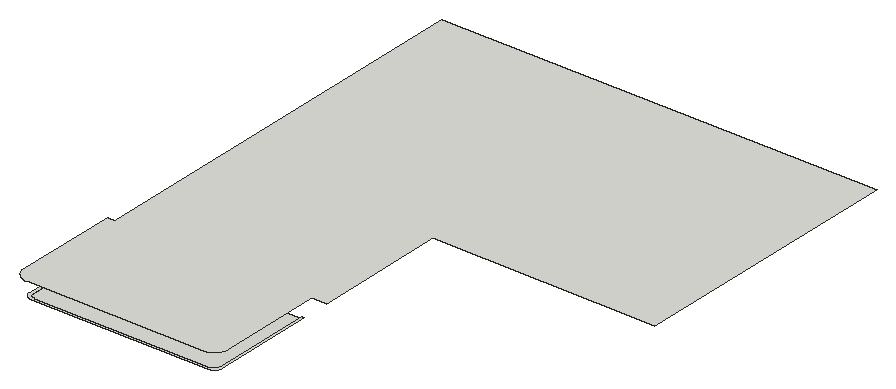
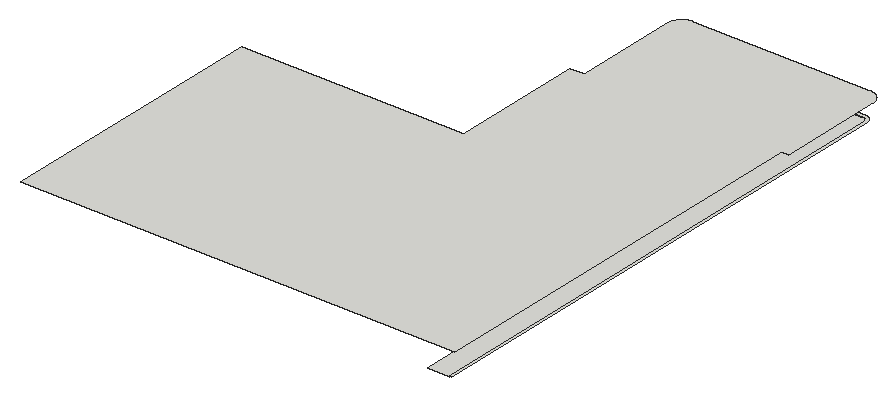
# SketchUp Ruby script. Lengths in inches.
U = 1.inch
M = Sketchup.active_model
def pt(a) = Geom::Point3d.new(a.map { |v| v * U })
def face(e, loops, mat)
  f = e.add_face(loops[0].map { |a| pt(a) })
  loops[1..].each { |l| e.add_face(l.map { |a| pt(a) }).erase! }
  f.material = f.back_material = mat if mat
  f
end
# faces: each face lists its corners as indices into pts; further lists are holes
def faces(e, pts, list, mat = nil) = list.each { |f| face(e, (f[0].is_a?(Array) ? f : [f]).map { |l| l.map { |i| pts[i] } }, mat) }
# xy, xz, yz: faces in a plane at the given z, y or x. An outline is a flat list of corners, or four numbers for a rectangle; further outlines are holes
def ring(l) = l.size == 4 ? [[l[0], l[1]], [l[2], l[1]], [l[2], l[3]], [l[0], l[3]]] : l.each_slice(2).to_a
def flat(e, list, mat, &to3) = list.each { |f| face(e, (f[0].is_a?(Array) ? f : [f]).map { |l| ring(l).map { |u, v| to3.(u, v) } }, mat) }
def xy(e, z, list, mat = nil) = flat(e, list, mat) { |x, y| [x, y, z] }
def xz(e, y, list, mat = nil) = flat(e, list, mat) { |x, z| [x, y, z] }
def yz(e, x, list, mat = nil) = flat(e, list, mat) { |y, z| [x, y, z] }
def lines(e, pts, list) = list.each { |a, b| e.add_line(pt(pts[a]), pt(pts[b])) }
# prism: a flat outline (further loops are holes) pulled along v
def prism(e, loops, v, mat = nil)
  f = face(e, loops, mat); d = Geom::Vector3d.new(v.map { |x| x * U })
  f.pushpull(f.normal.samedirection?(d) ? d.length : -d.length)
end
def box(e, o, s, mat = nil) = prism(e, [[o, [o[0] + s[0], o[1], o[2]], [o[0] + s[0], o[1] + s[1], o[2]], [o[0], o[1] + s[1], o[2]]]], [0, 0, s[2]], mat)
def at(x, y, z, deg = 0) = Geom::Transformation.translation(pt([x, y, z])) * Geom::Transformation.rotation(ORIGIN, Z_AXIS, deg.degrees)
def axes(o, x, y, z) = Geom::Transformation.new([*x, 0, *y, 0, *z, 0, *pt(o).to_a, 1])
def part(name) = M.definitions.add(name)
# library, detail: a bought-in or finely detailed component or shape, given as its bounding box
def library(name, o, s) = part(name).tap { |d| box(d.entities, o, s) }
def detail(e, o, s) = box(e.add_group.entities, o, s)
def put(e, d, t, mat = nil) = e.add_instance(d, t).tap { |i| i.material = mat if mat }
def group(e, t, mat = nil) = e.add_group.tap { |g| g.transformation = t; g.material = mat if mat }.entities
root = M.entities
xy(root,247,[[[29.8,234,29.74,234.01,29.67,234.01,29.61,234.02,29.54,234.02,29.48,234.03,29.41,234.03,29.35,234.04,29.28,234.05,29.22,234.0625,29.15,234.07,29.09,234.08,29.02,234.1,28.96,234.11,28.9,234.125,28.83,234.14,28.77,234.15,28.71,234.17,28.64,234.1875,28.58,234.21,28.52,234.22,28.45,234.24,28.39,234.27,28.21,234.33,28.15,234.36,28.09,234.38,28.03,234.41,27.97,234.43,27.79,234.52,27.73,234.54,27.67,234.58,27.61,234.61,27.56,234.64,27.44,234.7,27.39,234.74,27.33,234.77,27.28,234.81,27.22,234.84,27.17,234.88,27.11,234.92,27.0625,234.95,27.01,234.99,26.96,235.03,26.9,235.07,26.85,235.11,26.8,235.16,26.65,235.28,26.61,235.33,26.51,235.42,26.46,235.46,26.42,235.51,26.33,235.61,26.28,235.65,26.16,235.8,26.11,235.85,26.07,235.9,26.03,235.96,25.99,236.01,25.95,236.0625,25.92,236.11,25.88,236.17,25.84,236.22,25.81,236.28,25.77,236.33,25.74,236.39,25.7,236.44,25.64,236.56,25.61,236.61,25.58,236.67,25.54,236.73,25.52,236.79,25.43,236.97,25.41,237.03,25.38,237.09,25.36,237.15,25.33,237.21,25.27,237.39,25.24,237.45,25.22,237.52,25.21,237.58,25.1875,237.64,25.17,237.71,25.15,237.77,25.14,237.83,25.125,237.9,25.11,237.96,25.1,238.02,25.08,238.09,25.07,238.15,25.0625,238.22,25.05,238.28,25.04,238.35,25.03,238.41,25.03,238.48,25.02,238.54,25.02,238.61,25.01,238.67,25.01,238.74,25,238.8,25,672,43,672,43,323.75,182,323.75,182,238.8,181.99,238.74,181.99,238.67,181.98,238.61,181.98,238.54,181.97,238.48,181.97,238.41,181.96,238.35,181.95,238.28,181.9375,238.22,181.93,238.15,181.92,238.09,181.9,238.02,181.89,237.96,181.875,237.9,181.86,237.83,181.85,237.77,181.83,237.71,181.8125,237.64,181.79,237.58,181.78,237.52,181.76,237.45,181.73,237.39,181.67,237.21,181.64,237.15,181.62,237.09,181.59,237.03,181.57,236.97,181.48,236.79,181.46,236.73,181.42,236.67,181.39,236.61,181.36,236.56,181.3,236.44,181.26,236.39,181.23,236.33,181.19,236.28,181.16,236.22,181.12,236.17,181.08,236.11,181.05,236.0625,181.01,236.01,180.97,235.96,180.93,235.9,180.89,235.85,180.84,235.8,180.72,235.65,180.67,235.61,180.58,235.51,180.54,235.46,180.49,235.42,180.39,235.33,180.35,235.28,180.2,235.16,180.15,235.11,180.1,235.07,180.04,235.03,179.99,234.99,179.9375,234.95,179.89,234.92,179.83,234.88,179.78,234.84,179.72,234.81,179.67,234.77,179.61,234.74,179.56,234.7,179.44,234.64,179.39,234.61,179.33,234.58,179.27,234.54,179.21,234.52,179.03,234.43,178.97,234.41,178.91,234.38,178.85,234.36,178.79,234.33,178.61,234.27,178.55,234.24,178.48,234.22,178.42,234.21,178.36,234.1875,178.29,234.17,178.23,234.15,178.17,234.14,178.1,234.125,178.04,234.11,177.98,234.1,177.91,234.08,177.85,234.07,177.78,234.0625,177.72,234.05,177.65,234.04,177.59,234.03,177.52,234.03,177.46,234.02,177.39,234.02,177.33,234.01,177.26,234.01,177.2,234],[103.34,272.75,103.66,272.75,103.74,272.76,103.8125,272.77,103.89,272.78,104.05,272.8,104.125,272.82,104.2,272.83,104.28,272.85,104.35,272.875,104.43,272.9,104.5,272.92,104.58,272.95,104.79,273.04,104.86,273.08,104.93,273.11,105.07,273.19,105.13,273.23,105.2,273.28,105.26,273.32,105.33,273.37,105.57,273.57,105.62,273.63,105.68,273.68,105.88,273.92,105.93,273.99,105.97,274.05,106.02,274.12,106.06,274.18,106.14,274.32,106.17,274.39,106.21,274.46,106.3,274.67,106.33,274.75,106.35,274.82,106.375,274.9,106.4,274.97,106.42,275.05,106.43,275.125,106.45,275.2,106.47,275.36,106.48,275.4375,106.49,275.51,106.5,275.59,106.5,275.91,106.49,275.99,106.48,276.0625,106.47,276.14,106.45,276.3,106.43,276.375,106.42,276.45,106.4,276.53,106.375,276.6,106.35,276.68,106.33,276.75,106.3,276.83,106.21,277.04,106.17,277.11,106.14,277.18,106.06,277.32,106.02,277.38,105.97,277.45,105.93,277.51,105.88,277.58,105.68,277.82,105.62,277.87,105.57,277.93,105.33,278.13,105.26,278.18,105.2,278.22,105.13,278.27,105.07,278.31,104.93,278.39,104.86,278.42,104.79,278.46,104.58,278.55,104.5,278.58,104.43,278.6,104.35,278.625,104.28,278.65,104.2,278.67,104.125,278.68,104.05,278.7,103.89,278.72,103.8125,278.73,103.74,278.74,103.66,278.75,103.34,278.75,103.26,278.74,103.1875,278.73,103.11,278.72,102.95,278.7,102.875,278.68,102.8,278.67,102.72,278.65,102.65,278.625,102.57,278.6,102.5,278.58,102.42,278.55,102.21,278.46,102.14,278.42,102.07,278.39,101.93,278.31,101.87,278.27,101.8,278.22,101.74,278.18,101.67,278.13,101.43,277.93,101.38,277.87,101.32,277.82,101.12,277.58,101.07,277.51,101.03,277.45,100.98,277.38,100.94,277.32,100.86,277.18,100.83,277.11,100.79,277.04,100.7,276.83,100.67,276.75,100.65,276.68,100.625,276.6,100.6,276.53,100.58,276.45,100.57,276.375,100.55,276.3,100.53,276.14,100.52,276.0625,100.51,275.99,100.5,275.91,100.5,275.59,100.51,275.51,100.52,275.4375,100.53,275.36,100.55,275.2,100.57,275.125,100.58,275.05,100.6,274.97,100.625,274.9,100.65,274.82,100.67,274.75,100.7,274.67,100.79,274.46,100.83,274.39,100.86,274.32,100.94,274.18,100.98,274.12,101.03,274.05,101.07,273.99,101.12,273.92,101.32,273.68,101.38,273.63,101.43,273.57,101.67,273.37,101.74,273.32,101.8,273.28,101.87,273.23,101.93,273.19,102.07,273.11,102.14,273.08,102.21,273.04,102.42,272.95,102.5,272.92,102.57,272.9,102.65,272.875,102.72,272.85,102.8,272.83,102.875,272.82,102.95,272.8,103.11,272.78,103.1875,272.77,103.26,272.76],[150.79,272.75,151.1,272.75,151.34,272.78,151.41,272.79,151.49,272.8,151.57,272.82,151.65,272.83,151.72,272.85,151.8,272.875,151.87,272.9,151.95,272.92,152.09,272.98,152.17,273.01,152.24,273.04,152.31,273.08,152.375,273.11,152.45,273.15,152.51,273.19,152.58,273.23,152.64,273.28,152.71,273.32,153.01,273.57,153.12,273.68,153.17,273.74,153.23,273.8,153.33,273.92,153.37,273.99,153.42,274.05,153.46,274.12,153.5,274.18,153.62,274.39,153.65,274.46,153.6875,274.53,153.72,274.6,153.75,274.67,153.77,274.75,153.8,274.82,153.82,274.9,153.84,274.97,153.86,275.05,153.88,275.125,153.89,275.2,153.91,275.28,153.92,275.36,153.93,275.4375,153.9375,275.51,153.94,275.59,153.94,275.67,153.95,275.75,153.94,275.83,153.94,275.91,153.9375,275.99,153.93,276.0625,153.92,276.14,153.91,276.22,153.89,276.3,153.88,276.375,153.86,276.45,153.84,276.53,153.82,276.6,153.8,276.68,153.77,276.75,153.75,276.83,153.72,276.9,153.6875,276.97,153.65,277.04,153.62,277.11,153.5,277.32,153.46,277.38,153.42,277.45,153.37,277.51,153.33,277.58,153.23,277.7,153.17,277.76,153.12,277.82,153.01,277.93,152.71,278.18,152.64,278.22,152.58,278.27,152.51,278.31,152.45,278.35,152.375,278.39,152.31,278.42,152.24,278.46,152.17,278.49,152.09,278.52,151.95,278.58,151.87,278.6,151.8,278.625,151.72,278.65,151.65,278.67,151.57,278.68,151.49,278.7,151.41,278.71,151.34,278.72,151.1,278.75,150.79,278.75,150.55,278.72,150.48,278.71,150.4,278.7,150.32,278.68,150.24,278.67,150.17,278.65,150.09,278.625,150.02,278.6,149.94,278.58,149.73,278.49,149.65,278.46,149.58,278.42,149.51,278.39,149.45,278.35,149.38,278.31,149.3125,278.27,149.25,278.22,149.18,278.18,149,278.03,148.9375,277.98,148.88,277.93,148.77,277.82,148.72,277.76,148.66,277.7,148.61,277.64,148.57,277.58,148.52,277.51,148.47,277.45,148.43,277.38,148.39,277.32,148.27,277.11,148.24,277.04,148.2,276.97,148.14,276.83,148.12,276.75,148.09,276.68,148.07,276.6,148.05,276.53,148.03,276.45,148.01,276.375,148,276.3,147.98,276.22,147.97,276.14,147.96,276.0625,147.95,275.99,147.95,275.51,147.96,275.4375,147.97,275.36,147.98,275.28,148,275.2,148.01,275.125,148.03,275.05,148.05,274.97,148.07,274.9,148.09,274.82,148.12,274.75,148.14,274.67,148.2,274.53,148.24,274.46,148.27,274.39,148.39,274.18,148.43,274.12,148.47,274.05,148.52,273.99,148.57,273.92,148.61,273.86,148.66,273.8,148.72,273.74,148.77,273.68,148.88,273.57,148.9375,273.52,149,273.47,149.18,273.32,149.25,273.28,149.3125,273.23,149.38,273.19,149.45,273.15,149.51,273.11,149.58,273.08,149.65,273.04,149.73,273.01,149.94,272.92,150.02,272.9,150.09,272.875,150.17,272.85,150.24,272.83,150.32,272.82,150.4,272.8,150.48,272.79,150.55,272.78],[55.9,272.75,56.21,272.75,56.45,272.78,56.52,272.79,56.6,272.8,56.68,272.82,56.76,272.83,56.83,272.85,56.91,272.875,56.98,272.9,57.06,272.92,57.27,273.01,57.35,273.04,57.42,273.08,57.49,273.11,57.55,273.15,57.62,273.19,57.6875,273.23,57.75,273.28,57.82,273.32,58,273.47,58.0625,273.52,58.12,273.57,58.23,273.68,58.28,273.74,58.34,273.8,58.39,273.86,58.43,273.92,58.48,273.99,58.53,274.05,58.57,274.12,58.61,274.18,58.73,274.39,58.76,274.46,58.8,274.53,58.86,274.67,58.88,274.75,58.91,274.82,58.93,274.9,58.95,274.97,58.97,275.05,58.99,275.125,59,275.2,59.02,275.28,59.03,275.36,59.04,275.4375,59.05,275.51,59.05,275.99,59.04,276.0625,59.03,276.14,59.02,276.22,59,276.3,58.99,276.375,58.97,276.45,58.95,276.53,58.93,276.6,58.91,276.68,58.88,276.75,58.86,276.83,58.8,276.97,58.76,277.04,58.73,277.11,58.61,277.32,58.57,277.38,58.53,277.45,58.48,277.51,58.43,277.58,58.39,277.64,58.34,277.7,58.28,277.76,58.23,277.82,58.12,277.93,58.0625,277.98,58,278.03,57.82,278.18,57.75,278.22,57.6875,278.27,57.62,278.31,57.55,278.35,57.49,278.39,57.42,278.42,57.35,278.46,57.27,278.49,57.06,278.58,56.98,278.6,56.91,278.625,56.83,278.65,56.76,278.67,56.68,278.68,56.6,278.7,56.52,278.71,56.45,278.72,56.21,278.75,55.9,278.75,55.66,278.72,55.59,278.71,55.51,278.7,55.43,278.68,55.35,278.67,55.28,278.65,55.2,278.625,55.13,278.6,55.05,278.58,54.91,278.52,54.83,278.49,54.76,278.46,54.69,278.42,54.625,278.39,54.55,278.35,54.49,278.31,54.42,278.27,54.36,278.22,54.29,278.18,53.99,277.93,53.88,277.82,53.83,277.76,53.77,277.7,53.67,277.58,53.63,277.51,53.58,277.45,53.54,277.38,53.5,277.32,53.38,277.11,53.35,277.04,53.3125,276.97,53.28,276.9,53.25,276.83,53.23,276.75,53.2,276.68,53.18,276.6,53.16,276.53,53.14,276.45,53.12,276.375,53.11,276.3,53.09,276.22,53.08,276.14,53.07,276.0625,53.0625,275.99,53.06,275.91,53.06,275.83,53.05,275.75,53.06,275.67,53.06,275.59,53.0625,275.51,53.07,275.4375,53.08,275.36,53.09,275.28,53.11,275.2,53.12,275.125,53.14,275.05,53.16,274.97,53.18,274.9,53.2,274.82,53.23,274.75,53.25,274.67,53.28,274.6,53.3125,274.53,53.35,274.46,53.38,274.39,53.5,274.18,53.54,274.12,53.58,274.05,53.63,273.99,53.67,273.92,53.77,273.8,53.83,273.74,53.88,273.68,53.99,273.57,54.29,273.32,54.36,273.28,54.42,273.23,54.49,273.19,54.55,273.15,54.625,273.11,54.69,273.08,54.76,273.04,54.83,273.01,54.91,272.98,55.05,272.92,55.13,272.9,55.2,272.875,55.28,272.85,55.35,272.83,55.43,272.82,55.51,272.8,55.59,272.79,55.66,272.78]]])
xy(root,248,[[29.82,232,29.73,232.01,29.54,232.01,29,232.07,28.9,232.09,28.81,232.1,28.72,232.12,28.63,232.13,28.54,232.15,28.46,232.17,28.37,232.19,28.28,232.22,28.1875,232.24,28.1,232.26,28.01,232.29,27.92,232.31,27.84,232.34,27.66,232.4,27.58,232.43,27.49,232.46,27.41,232.5,27.32,232.53,27.24,232.57,27.15,232.61,27.07,232.64,26.99,232.68,26.9,232.72,26.82,232.76,26.74,232.81,26.58,232.89,26.5,232.9375,26.42,232.98,26.26,233.08,26.1875,233.13,26.11,233.18,26.04,233.23,25.96,233.28,25.89,233.34,25.8125,233.39,25.74,233.45,25.67,233.5,25.59,233.56,25.38,233.74,25.32,233.8,25.18,233.92,25.12,233.99,25.05,234.05,24.99,234.12,24.92,234.18,24.8,234.32,24.74,234.38,24.56,234.59,24.5,234.67,24.45,234.74,24.39,234.8125,24.34,234.89,24.28,234.96,24.23,235.04,24.18,235.11,24.13,235.1875,24.08,235.26,23.98,235.42,23.9375,235.5,23.89,235.58,23.81,235.74,23.76,235.82,23.72,235.9,23.68,235.99,23.64,236.07,23.61,236.15,23.57,236.24,23.53,236.32,23.5,236.41,23.46,236.49,23.43,236.58,23.4,236.66,23.34,236.84,23.31,236.92,23.29,237.01,23.26,237.1,23.24,237.1875,23.22,237.28,23.19,237.37,23.17,237.46,23.15,237.54,23.13,237.63,23.12,237.72,23.1,237.81,23.09,237.9,23.07,238,23.01,238.54,23.01,238.73,23,238.82,23,672,25,672,25,238.8,25.01,238.74,25.01,238.67,25.02,238.61,25.02,238.54,25.03,238.48,25.03,238.41,25.04,238.35,25.05,238.28,25.0625,238.22,25.07,238.15,25.08,238.09,25.1,238.02,25.11,237.96,25.125,237.9,25.14,237.83,25.15,237.77,25.17,237.71,25.1875,237.64,25.21,237.58,25.22,237.52,25.24,237.45,25.27,237.39,25.33,237.21,25.36,237.15,25.38,237.09,25.41,237.03,25.43,236.97,25.52,236.79,25.54,236.73,25.58,236.67,25.61,236.61,25.64,236.56,25.7,236.44,25.74,236.39,25.77,236.33,25.81,236.28,25.84,236.22,25.88,236.17,25.92,236.11,25.95,236.0625,25.99,236.01,26.03,235.96,26.07,235.9,26.11,235.85,26.16,235.8,26.28,235.65,26.33,235.61,26.42,235.51,26.46,235.46,26.51,235.42,26.61,235.33,26.65,235.28,26.8,235.16,26.85,235.11,26.9,235.07,26.96,235.03,27.01,234.99,27.0625,234.95,27.11,234.92,27.17,234.88,27.22,234.84,27.28,234.81,27.33,234.77,27.39,234.74,27.44,234.7,27.56,234.64,27.61,234.61,27.67,234.58,27.73,234.54,27.79,234.52,27.97,234.43,28.03,234.41,28.09,234.38,28.15,234.36,28.21,234.33,28.39,234.27,28.45,234.24,28.52,234.22,28.58,234.21,28.64,234.1875,28.71,234.17,28.77,234.15,28.83,234.14,28.9,234.125,28.96,234.11,29.02,234.1,29.09,234.08,29.15,234.07,29.22,234.0625,29.28,234.05,29.35,234.04,29.41,234.03,29.48,234.03,29.54,234.02,29.61,234.02,29.67,234.01,29.74,234.01,29.8,234,177.2,234,177.26,234.01,177.33,234.01,177.39,234.02,177.46,234.02,177.52,234.03,177.59,234.03,177.65,234.04,177.72,234.05,177.78,234.0625,177.85,234.07,177.91,234.08,177.98,234.1,178.04,234.11,178.1,234.125,178.17,234.14,178.23,234.15,178.29,234.17,178.36,234.1875,178.42,234.21,178.48,234.22,178.55,234.24,178.61,234.27,178.79,234.33,178.85,234.36,178.91,234.38,178.97,234.41,179.03,234.43,179.21,234.52,179.27,234.54,179.33,234.58,179.39,234.61,179.44,234.64,179.56,234.7,179.61,234.74,179.67,234.77,179.72,234.81,179.78,234.84,179.83,234.88,179.89,234.92,179.9375,234.95,179.99,234.99,180.04,235.03,180.1,235.07,180.15,235.11,180.2,235.16,180.35,235.28,180.39,235.33,180.49,235.42,180.54,235.46,180.58,235.51,180.67,235.61,180.72,235.65,180.84,235.8,180.89,235.85,180.93,235.9,180.97,235.96,181.01,236.01,181.05,236.0625,181.08,236.11,181.12,236.17,181.16,236.22,181.19,236.28,181.23,236.33,181.26,236.39,181.3,236.44,181.36,236.56,181.39,236.61,181.42,236.67,181.46,236.73,181.48,236.79,181.57,236.97,181.59,237.03,181.62,237.09,181.64,237.15,181.67,237.21,181.73,237.39,181.76,237.45,181.78,237.52,181.79,237.58,181.8125,237.64,181.83,237.71,181.85,237.77,181.86,237.83,181.875,237.9,181.89,237.96,181.9,238.02,181.92,238.09,181.93,238.15,181.9375,238.22,181.95,238.28,181.96,238.35,181.97,238.41,181.97,238.48,181.98,238.54,181.98,238.61,181.99,238.67,181.99,238.74,182,238.8,182,323.75,184,323.75,184,238.82,183.99,238.73,183.99,238.54,183.93,238,183.91,237.9,183.9,237.81,183.88,237.72,183.87,237.63,183.85,237.54,183.83,237.46,183.81,237.37,183.78,237.28,183.76,237.1875,183.74,237.1,183.71,237.01,183.69,236.92,183.66,236.84,183.6,236.66,183.57,236.58,183.54,236.49,183.5,236.41,183.47,236.32,183.43,236.24,183.39,236.15,183.36,236.07,183.32,235.99,183.28,235.9,183.24,235.82,183.19,235.74,183.11,235.58,183.0625,235.5,183.02,235.42,182.92,235.26,182.87,235.1875,182.82,235.11,182.77,235.04,182.72,234.96,182.66,234.89,182.61,234.8125,182.55,234.74,182.5,234.67,182.44,234.59,182.26,234.38,182.2,234.32,182.08,234.18,182.01,234.12,181.95,234.05,181.88,233.99,181.82,233.92,181.68,233.8,181.62,233.74,181.41,233.56,181.33,233.5,181.26,233.45,181.1875,233.39,181.11,233.34,181.04,233.28,180.96,233.23,180.89,233.18,180.8125,233.13,180.74,233.08,180.58,232.98,180.5,232.9375,180.42,232.89,180.26,232.81,180.18,232.76,180.1,232.72,180.01,232.68,179.93,232.64,179.85,232.61,179.76,232.57,179.68,232.53,179.59,232.5,179.51,232.46,179.42,232.43,179.34,232.4,179.16,232.34,179.08,232.31,178.99,232.29,178.9,232.26,178.8125,232.24,178.72,232.22,178.63,232.19,178.54,232.17,178.46,232.15,178.37,232.13,178.28,232.12,178.19,232.1,178.1,232.09,178,232.07,177.46,232.01,177.27,232.01,177.18,232]])
xy(root,264,[[29.6875,227,177.3125,227,177.47,227.01,177.63,227.02,177.78,227.03,178.1,227.05,178.25,227.07,178.41,227.08,178.57,227.1,178.72,227.125,178.88,227.15,179.03,227.17,179.1875,227.2,179.34,227.23,179.49,227.26,179.65,227.3,179.8,227.33,179.95,227.37,180.11,227.41,180.41,227.49,180.86,227.64,181.01,227.6875,181.15,227.74,181.3,227.8,181.45,227.85,181.59,227.91,181.74,227.97,181.88,228.04,182.02,228.1,182.17,228.17,182.73,228.45,182.86,228.53,183,228.61,183.14,228.6875,183.27,228.77,183.4,228.85,183.54,228.9375,183.67,229.02,183.93,229.2,184.05,229.29,184.18,229.38,184.31,229.48,184.43,229.58,184.55,229.67,184.67,229.77,184.91,229.98,185.03,230.08,185.15,230.1875,185.26,230.3,185.375,230.4,185.49,230.51,185.6,230.625,185.7,230.74,185.8125,230.85,185.92,230.97,186.02,231.09,186.23,231.33,186.33,231.45,186.42,231.57,186.52,231.69,186.62,231.82,186.71,231.95,186.8,232.07,186.98,232.33,187.0625,232.46,187.15,232.6,187.23,232.73,187.3125,232.86,187.39,233,187.47,233.14,187.55,233.27,187.83,233.83,187.9,233.98,187.96,234.12,188.03,234.26,188.09,234.41,188.15,234.55,188.2,234.7,188.26,234.85,188.3125,234.99,188.36,235.14,188.51,235.59,188.59,235.89,188.63,236.05,188.67,236.2,188.7,236.35,188.74,236.51,188.77,236.66,188.8,236.8125,188.83,236.97,188.85,237.12,188.875,237.28,188.9,237.43,188.92,237.59,188.93,237.75,188.95,237.9,188.97,238.22,188.98,238.37,188.99,238.53,189,238.6875,189,326,201,326,201,437,387,437,387,668,24,668,24,326.09,18,326.09,18,238.6875,18.01,238.53,18.02,238.37,18.03,238.22,18.05,237.9,18.07,237.75,18.08,237.59,18.1,237.43,18.125,237.28,18.15,237.12,18.17,236.97,18.2,236.8125,18.23,236.66,18.26,236.51,18.3,236.35,18.33,236.2,18.37,236.05,18.41,235.89,18.49,235.59,18.64,235.14,18.6875,234.99,18.74,234.85,18.8,234.7,18.85,234.55,18.91,234.41,18.97,234.26,19.04,234.12,19.1,233.98,19.17,233.83,19.45,233.27,19.53,233.14,19.61,233,19.6875,232.86,19.77,232.73,19.85,232.6,19.9375,232.46,20.02,232.33,20.2,232.07,20.29,231.95,20.38,231.82,20.48,231.69,20.58,231.57,20.67,231.45,20.77,231.33,20.98,231.09,21.08,230.97,21.1875,230.85,21.3,230.74,21.4,230.625,21.51,230.51,21.625,230.4,21.74,230.3,21.85,230.1875,21.97,230.08,22.09,229.98,22.33,229.77,22.45,229.67,22.57,229.58,22.69,229.48,22.82,229.38,22.95,229.29,23.07,229.2,23.33,229.02,23.46,228.9375,23.6,228.85,23.73,228.77,23.86,228.6875,24,228.61,24.14,228.53,24.27,228.45,24.83,228.17,24.98,228.1,25.12,228.04,25.26,227.97,25.41,227.91,25.55,227.85,25.7,227.8,25.85,227.74,25.99,227.6875,26.14,227.64,26.59,227.49,26.89,227.41,27.05,227.37,27.2,227.33,27.35,227.3,27.51,227.26,27.66,227.23,27.8125,227.2,27.97,227.17,28.12,227.15,28.28,227.125,28.43,227.1,28.59,227.08,28.75,227.07,28.9,227.05,29.22,227.03,29.37,227.02,29.53,227.01]])
xz(root,272.75,[[103.34,247,103.42,250],[103.42,247,103.5,250],[103.5,247,103.58,250],[103.58,247,103.66,250],[150.79,247,150.87,250],
  [150.87,247,150.95,250],[150.95,247,151.02,250],[151.02,247,151.1,250]])
p = [[102.8,272.83,250],[102.8,272.83,247],[102.72,272.85,247],[102.72,272.85,250],[102.875,272.82,250],[102.875,272.82,247],
  [102.95,272.8,250],[102.95,272.8,247],[103.03,272.79,250],[103.03,272.79,247],[103.11,272.78,250],[103.11,272.78,247],
  [103.1875,272.77,250],[103.1875,272.77,247],[103.26,272.76,250],[103.26,272.76,247],[103.34,272.75,250],[103.34,272.75,247],
  [103.74,272.76,250],[103.74,272.76,247],[103.66,272.75,247],[103.66,272.75,250],[103.8125,272.77,250],[103.8125,272.77,247],
  [103.89,272.78,250],[103.89,272.78,247],[103.97,272.79,250],[103.97,272.79,247],[104.05,272.8,250],[104.05,272.8,247],
  [104.125,272.82,250],[104.125,272.82,247],[104.2,272.83,250],[104.2,272.83,247],[104.28,272.85,250],[104.28,272.85,247],
  [150.24,272.83,250],[150.24,272.83,247],[150.17,272.85,247],[150.17,272.85,250],[150.32,272.82,250],[150.32,272.82,247],
  [150.4,272.8,250],[150.4,272.8,247],[150.48,272.79,250],[150.48,272.79,247],[150.55,272.78,250],[150.55,272.78,247],
  [150.63,272.77,250],[150.63,272.77,247],[150.71,272.76,250],[150.71,272.76,247],[150.79,272.75,250],[150.79,272.75,247],
  [151.18,272.76,250],[151.18,272.76,247],[151.1,272.75,247],[151.1,272.75,250],[151.26,272.77,250],[151.26,272.77,247],
  [151.34,272.78,250],[151.34,272.78,247],[151.41,272.79,250],[151.41,272.79,247],[151.49,272.8,250],[151.49,272.8,247],
  [151.57,272.82,250],[151.57,272.82,247],[151.65,272.83,250],[151.65,272.83,247],[151.72,272.85,250],[151.72,272.85,247],
  [102.42,272.95,250],[102.42,272.95,247],[102.35,272.98,247],[102.35,272.98,250],[102.5,272.92,250],[102.5,272.92,247],
  [102.57,272.9,250],[102.57,272.9,247],[102.65,272.875,250],[102.65,272.875,247],[104.35,272.875,250],[104.35,272.875,247],
  [104.43,272.9,250],[104.43,272.9,247],[104.5,272.92,250],[104.5,272.92,247],[104.58,272.95,250],[104.58,272.95,247],
  [104.65,272.98,250],[104.65,272.98,247],[149.87,272.95,250],[149.87,272.95,247],[149.8,272.98,247],[149.8,272.98,250],
  [149.94,272.92,250],[149.94,272.92,247],[150.02,272.9,250],[150.02,272.9,247],[150.09,272.875,250],[150.09,272.875,247],
  [151.8,272.875,250],[151.8,272.875,247],[151.87,272.9,250],[151.87,272.9,247],[151.95,272.92,250],[151.95,272.92,247],
  [152.02,272.95,250],[152.02,272.95,247],[152.09,272.98,250],[152.09,272.98,247],[102.21,273.04,250],[102.21,273.04,247],
  [102.14,273.08,247],[102.14,273.08,250],[102.28,273.01,250],[102.28,273.01,247],[104.72,273.01,250],[104.72,273.01,247],
  [104.79,273.04,250],[104.79,273.04,247],[104.86,273.08,250],[104.86,273.08,247],[149.65,273.04,250],[149.65,273.04,247],
  [149.58,273.08,247],[149.58,273.08,250],[149.73,273.01,250],[149.73,273.01,247],[152.17,273.01,250],[152.17,273.01,247],
  [152.24,273.04,250],[152.24,273.04,247],[152.31,273.08,250],[152.31,273.08,247],[102.07,273.11,250],[102.07,273.11,247],
  [102,273.15,247],[102,273.15,250],[104.93,273.11,250],[104.93,273.11,247],[105,273.15,250],[105,273.15,247],
  [149.51,273.11,250],[149.51,273.11,247],[149.45,273.15,247],[149.45,273.15,250],[152.375,273.11,250],[152.375,273.11,247],
  [152.45,273.15,250],[152.45,273.15,247],[101.87,273.23,250],[101.87,273.23,247],[101.8,273.28,247],[101.8,273.28,250],
  [101.93,273.19,250],[101.93,273.19,247],[105.07,273.19,250],[105.07,273.19,247],[105.13,273.23,250],[105.13,273.23,247],
  [105.2,273.28,250],[105.2,273.28,247],[149.3125,273.23,250],[149.3125,273.23,247],[149.25,273.28,247],[149.25,273.28,250],
  [149.38,273.19,250],[149.38,273.19,247],[152.51,273.19,250],[152.51,273.19,247],[152.58,273.23,250],[152.58,273.23,247],
  [152.64,273.28,250],[152.64,273.28,247],[101.74,273.32,250],[101.74,273.32,247],[101.67,273.37,247],[101.67,273.37,250],
  [105.26,273.32,250],[105.26,273.32,247],[105.33,273.37,250],[105.33,273.37,247],[149.18,273.32,250],[149.18,273.32,247],
  [149.12,273.37,247],[149.12,273.37,250],[152.71,273.32,250],[152.71,273.32,247],[152.77,273.37,250],[152.77,273.37,247],
  [57.94,273.42,250],[57.94,273.42,247],[57.88,273.37,247],[57.88,273.37,250],[58,273.47,250],[58,273.47,247],
  [101.61,273.42,250],[101.61,273.42,247],[101.55,273.47,247],[101.55,273.47,250],[105.39,273.42,250],[105.39,273.42,247],
  [105.45,273.47,250],[105.45,273.47,247],[149.06,273.42,250],[149.06,273.42,247],[149,273.47,247],[149,273.47,250],
  [152.83,273.42,250],[152.83,273.42,247],[152.89,273.47,250],[152.89,273.47,247],[58.0625,273.52,250],[58.0625,273.52,247],
  [58.12,273.57,250],[58.12,273.57,247],[101.49,273.52,250],[101.49,273.52,247],[101.43,273.57,247],[101.43,273.57,250],
  [105.51,273.52,250],[105.51,273.52,247],[105.57,273.57,250],[105.57,273.57,247],[148.9375,273.52,250],[148.9375,273.52,247],
  [148.88,273.57,247],[148.88,273.57,250],[152.95,273.52,250],[152.95,273.52,247],[153.01,273.57,250],[153.01,273.57,247],
  [58.18,273.63,250],[58.18,273.63,247],[58.23,273.68,250],[58.23,273.68,247],[101.38,273.63,250],[101.38,273.63,247],
  [101.32,273.68,247],[101.32,273.68,250],[105.62,273.63,250],[105.62,273.63,247],[105.68,273.68,250],[105.68,273.68,247],
  [148.82,273.63,250],[148.82,273.63,247],[148.77,273.68,247],[148.77,273.68,250],[153.07,273.63,250],[153.07,273.63,247],
  [153.12,273.68,250],[153.12,273.68,247],[58.28,273.74,250],[58.28,273.74,247],[58.34,273.8,250],[58.34,273.8,247],
  [101.27,273.74,250],[101.27,273.74,247],[101.22,273.8,247],[101.22,273.8,250],[105.73,273.74,250],[105.73,273.74,247],
  [105.78,273.8,250],[105.78,273.8,247],[148.72,273.74,250],[148.72,273.74,247],[148.66,273.8,247],[148.66,273.8,250],
  [153.17,273.74,250],[153.17,273.74,247],[101.17,273.86,247],[101.17,273.86,250],[148.61,273.86,247],[148.61,273.86,250]]
faces(root,p,[[0,1,2,3],[4,5,1,0],[6,7,5,4],[8,9,7,6],[10,11,9,8],[12,13,11,10],[14,15,13,12],[16,17,15,14],
  [18,19,20,21],[22,23,19,18],[24,25,23,22],[26,27,25,24],[28,29,27,26],[30,31,29,28],[32,33,31,30],[34,35,33,32],
  [36,37,38,39],[40,41,37,36],[42,43,41,40],[44,45,43,42],[46,47,45,44],[48,49,47,46],[50,51,49,48],[52,53,51,50],
  [54,55,56,57],[58,59,55,54],[60,61,59,58],[62,63,61,60],[64,65,63,62],[66,67,65,64],[68,69,67,66],[70,71,69,68],
  [72,73,74,75],[76,77,73,72],[78,79,77,76],[80,81,79,78],[3,2,81,80],[82,83,35,34],[84,85,83,82],[86,87,85,84],
  [88,89,87,86],[90,91,89,88],[92,93,94,95],[96,97,93,92],[98,99,97,96],[100,101,99,98],[39,38,101,100],[102,103,71,70],
  [104,105,103,102],[106,107,105,104],[108,109,107,106],[110,111,109,108],[112,113,114,115],[116,117,113,112],[75,74,117,116],[118,119,91,90],
  [120,121,119,118],[122,123,121,120],[124,125,126,127],[128,129,125,124],[95,94,129,128],[130,131,111,110],[132,133,131,130],[134,135,133,132],
  [136,137,138,139],[115,114,137,136],[140,141,123,122],[142,143,141,140],[144,145,146,147],[127,126,145,144],[148,149,135,134],[150,151,149,148],
  [152,153,154,155],[156,157,153,152],[139,138,157,156],[158,159,143,142],[160,161,159,158],[162,163,161,160],[164,165,166,167],[168,169,165,164],
  [147,146,169,168],[170,171,151,150],[172,173,171,170],[174,175,173,172],[176,177,178,179],[155,154,177,176],[180,181,163,162],[182,183,181,180],
  [184,185,186,187],[167,166,185,184],[188,189,175,174],[190,191,189,188],[192,193,194,195],[196,197,193,192],[198,199,200,201],[179,178,199,198],
  [202,203,183,182],[204,205,203,202],[206,207,208,209],[187,186,207,206],[210,211,191,190],[212,213,211,210],[214,215,197,196],[216,217,215,214],
  [218,219,220,221],[201,200,219,218],[222,223,205,204],[224,225,223,222],[226,227,228,229],[209,208,227,226],[230,231,213,212],[232,233,231,230],
  [234,235,217,216],[236,237,235,234],[238,239,240,241],[221,220,239,238],[242,243,225,224],[244,245,243,242],[246,247,248,249],[229,228,247,246],
  [250,251,233,232],[252,253,251,250],[254,255,237,236],[256,257,255,254],[258,259,260,261],[241,240,259,258],[262,263,245,244],[264,265,263,262],
  [266,267,268,269],[249,248,267,266],[270,271,253,252],[261,260,272,273],[269,268,274,275]])
